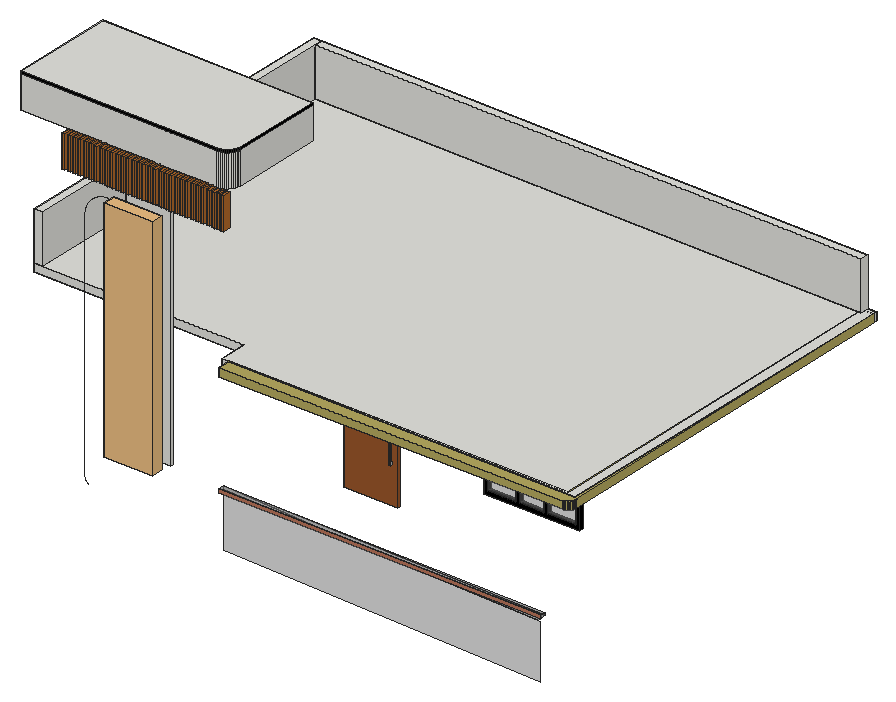
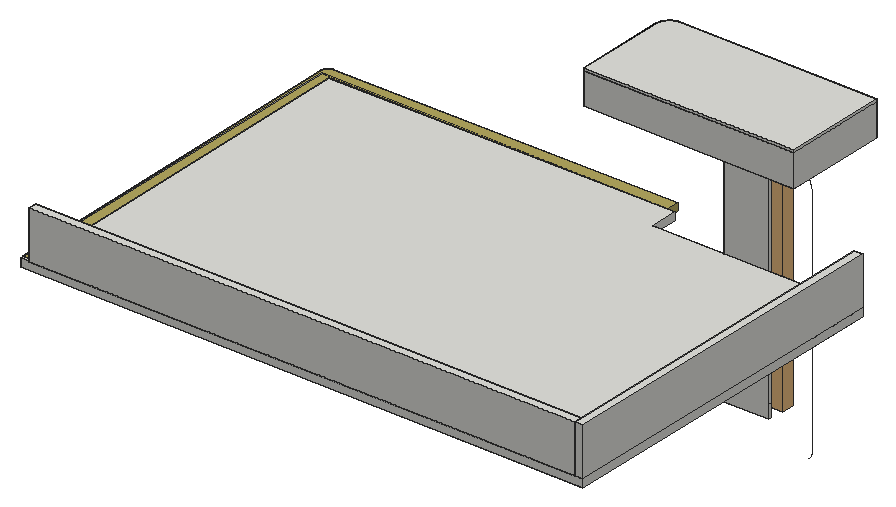
# SketchUp Ruby script. Lengths in inches.
U = 1.inch
M = Sketchup.active_model
def pt(a) = Geom::Point3d.new(a.map { |v| v * U })
def face(e, loops, mat)
  f = e.add_face(loops[0].map { |a| pt(a) })
  loops[1..].each { |l| e.add_face(l.map { |a| pt(a) }).erase! }
  f.material = f.back_material = mat if mat
  f
end
# faces: each face lists its corners as indices into pts; further lists are holes
def faces(e, pts, list, mat = nil) = list.each { |f| face(e, (f[0].is_a?(Array) ? f : [f]).map { |l| l.map { |i| pts[i] } }, mat) }
# xy, xz, yz: faces in a plane at the given z, y or x. An outline is a flat list of corners, or four numbers for a rectangle; further outlines are holes
def ring(l) = l.size == 4 ? [[l[0], l[1]], [l[2], l[1]], [l[2], l[3]], [l[0], l[3]]] : l.each_slice(2).to_a
def flat(e, list, mat, &to3) = list.each { |f| face(e, (f[0].is_a?(Array) ? f : [f]).map { |l| ring(l).map { |u, v| to3.(u, v) } }, mat) }
def xy(e, z, list, mat = nil) = flat(e, list, mat) { |x, y| [x, y, z] }
def xz(e, y, list, mat = nil) = flat(e, list, mat) { |x, z| [x, y, z] }
def yz(e, x, list, mat = nil) = flat(e, list, mat) { |y, z| [x, y, z] }
def lines(e, pts, list) = list.each { |a, b| e.add_line(pt(pts[a]), pt(pts[b])) }
# prism: a flat outline (further loops are holes) pulled along v
def prism(e, loops, v, mat = nil)
  f = face(e, loops, mat); d = Geom::Vector3d.new(v.map { |x| x * U })
  f.pushpull(f.normal.samedirection?(d) ? d.length : -d.length)
end
def box(e, o, s, mat = nil) = prism(e, [[o, [o[0] + s[0], o[1], o[2]], [o[0] + s[0], o[1] + s[1], o[2]], [o[0], o[1] + s[1], o[2]]]], [0, 0, s[2]], mat)
def at(x, y, z, deg = 0) = Geom::Transformation.translation(pt([x, y, z])) * Geom::Transformation.rotation(ORIGIN, Z_AXIS, deg.degrees)
def axes(o, x, y, z) = Geom::Transformation.new([*x, 0, *y, 0, *z, 0, *pt(o).to_a, 1])
def part(name) = M.definitions.add(name)
# library, detail: a bought-in or finely detailed component or shape, given as its bounding box
def library(name, o, s) = part(name).tap { |d| box(d.entities, o, s) }
def detail(e, o, s) = box(e.add_group.entities, o, s)
def put(e, d, t, mat = nil) = e.add_instance(d, t).tap { |i| i.material = mat if mat }
def group(e, t, mat = nil) = e.add_group.tap { |g| g.transformation = t; g.material = mat if mat }.entities
root = M.entities
M.materials.add("[Aluminum]").color = [179, 179, 179]
M.materials.add("[Color M06]").color = [86, 86, 86]
M.materials.add("[Color M09]").color = [0, 0, 0]
M.materials.add("[Metal Rusted]").color = [184, 117, 91]
M.materials.add("[Translucent Glass Gray]").color = [128, 128, 128]
M.materials["[Translucent Glass Gray]"].alpha = 0.5
M.materials.add("[Wood Bamboo]").color = [177, 105, 43]
M.materials.add("[Wood Board Cork]").color = [181, 169, 96]
M.materials.add("[Wood Cherry Original]").color = [152, 86, 42]
c1 = part("Group\#8")
box(c1.entities,[0,-2,0],[40,2,76])
c2 = part("Group\#13")
prism(c2.entities,[[[1.25,1.5,24.92],[1.25,1.5,26.5625],[1.25,0,26.5625],[1.25,0,0],[1.25,1.5,0],[1.25,1.5,1.64],[1.25,0.64,1.64],[1.25,0.64,24.92]]],[-1.25,0,0])
c3 = part("Group\#3")
prism(c3.entities,[[[0,3,0],[0,3,48],[72,3,48],[72,3,0]],[[24,3,3],[24,3,45],[3,3,45],[3,3,3]],[[69,3,45],[48,3,45],[48,3,3],[69,3,3]],[[45,3,3],[45,3,45],[27,3,45],[27,3,3]]],[0,-3,0])
c4 = part("Group\#6")
xz(c4.entities,0,[[0,0,21,42]])
c5 = part("Group\#5")
xz(c5.entities,0,[[0,0,18,42]])
c6 = part("Group\#4")
xz(c6.entities,0,[[0,0,21,42]])
c7 = part("Group\#33")
box(c7.entities,[0,0,0],[2.28,6,24])
xy(root,366,[[0,94.33,0,171.62,156.72,171.62,156.72,104.31,156.64,103.01,156.38,101.73,155.96,100.49,155.39,99.32,154.66,98.24,153.8,97.26,152.82,96.39,151.73,95.67,150.5625,95.09,149.33,94.67,148.05,94.42,146.75,94.33]])
xy(root,390,[[0,94.33,146.75,94.33,148.05,94.42,149.33,94.67,150.5625,95.09,151.73,95.67,152.82,96.39,153.8,97.26,154.66,98.24,155.39,99.32,155.96,100.49,156.38,101.73,156.64,103.01,156.72,104.31,156.72,171.62,0,171.62]])
xy(root,392,[[0,94.33,146.75,94.33,148.05,94.42,149.33,94.67,150.5625,95.09,151.73,95.67,152.82,96.39,153.8,97.26,154.66,98.24,155.39,99.32,155.96,100.49,156.38,101.73,156.64,103.01,156.72,104.31,156.72,171.62,0,171.62]])
xz(root,94.33,[[0,366,146.75,390]])
xz(root,94.33,[[0,390,146.75,392]],"[Color M09]")
xz(root,171.62,[[0,366,156.72,390],[0,390,156.72,392]])
yz(root,0,[[94.33,366,171.62,390],[94.33,390,171.62,392]])
yz(root,156.72,[[104.31,366,171.62,390]])
yz(root,156.72,[[104.31,390,171.62,392]],"[Color M09]")
p = [[148.05,94.42,390],[146.75,94.33,390],[146.75,94.33,366],[148.05,94.42,366],[149.33,94.67,390],[149.33,94.67,366],
  [150.5625,95.09,390],[150.5625,95.09,366],[151.73,95.67,390],[151.73,95.67,366],[152.82,96.39,390],[152.82,96.39,366],
  [153.8,97.26,390],[153.8,97.26,366],[154.66,98.24,390],[154.66,98.24,366],[155.39,99.32,390],[155.39,99.32,366],
  [155.96,100.49,390],[155.96,100.49,366],[156.38,101.73,390],[156.38,101.73,366],[156.64,103.01,390],[156.64,103.01,366],
  [156.72,104.31,390],[156.72,104.31,366],[148.05,94.42,392],[146.75,94.33,392],[149.33,94.67,392],[150.5625,95.09,392],
  [151.73,95.67,392],[152.82,96.39,392],[153.8,97.26,392],[154.66,98.24,392],[155.39,99.32,392],[155.96,100.49,392],
  [156.38,101.73,392],[156.64,103.01,392],[156.72,104.31,392],[51.2,94.33,132.96],[50.6,94.33,133.37],[50.06,94.33,133.84],
  [49.5625,94.33,134.36],[49.13,94.33,134.94],[48.76,94.33,135.5625],[48.46,94.33,136.22],[48.24,94.33,136.9],[48.01,94.33,138.62],
  [48.01,94.33,312.18],[48.17,94.33,314.5],[48.62,94.33,316.79],[49.37,94.33,319],[50.4,94.33,321.09],[51.7,94.33,323.03],
  [53.23,94.33,324.78],[54.99,94.33,326.32],[56.93,94.33,327.61],[59.02,94.33,328.64],[61.22,94.33,329.39],[63.51,94.33,329.85],
  [65.84,94.33,330]]
faces(root,p,[[0,1,2,3],[4,0,3,5],[6,4,5,7],[8,6,7,9],[10,8,9,11],[12,10,11,13],[14,12,13,15],[16,14,15,17],
  [18,16,17,19],[20,18,19,21],[22,20,21,23],[24,22,23,25]])
faces(root,p,[[1,0,26,27],[0,4,28,26],[4,6,29,28],[6,8,30,29],[8,10,31,30],[10,12,32,31],[12,14,33,32],[14,16,34,33],
  [16,18,35,34],[18,20,36,35],[20,22,37,36],[22,24,38,37]],"[Color M09]")
lines(root,p,[[39,40],[40,41],[41,42],[42,43],[43,44],[44,45],[45,46],[47,48],[47,46],[48,49],[49,50],[50,51],
  [51,52],[52,53],[53,54],[54,55],[55,56],[56,57],[57,58],[58,59],[59,60]])
g1 = group(root,at(162.16,74.66,133.26),"[Translucent Glass Gray]")
xy(g1,40.75,[[241,0.04,241,2.61,0,2.61,0,6.79,104.85,3.86,149.47,2.61],[241,0.04,149.47,2.61,241,2.61],[149.47,2.61,104.85,3.86,241,6.79,241,2.61]])
xy(g1,43.375,[[0,2.61,241,6.79]])
xz(g1,2.61,[[0,40.75,241,43.375]],"[Metal Rusted]")
xz(g1,6.79,[[241,40.75,0,43.375,241,43.375]])
yz(g1,0,[[2.61,40.75,6.79,43.375]])
yz(g1,241,[[2.61,40.75,6.79,43.375]])
p = [[0,6.79,0],[0,6.79,40.75],[104.85,3.86,40.75],[149.47,2.61,40.75],[241,0.04,40.75],[242.54,0,40.75],
  [242.54,0,0],[0,6.79,43.375],[241,6.79,40.75]]
faces(g1,p,[[0,1,2,3,4,5,6],[1,7,2],[8,2,7]])
put(root,c1,at(172.72,182.76,136),"[Wood Cherry Original]")
g2 = group(root,at(69.91,107.39,158.71))
prism(g2,[[[0.09,0,10.1875],[0,0,10.1875],[0,0,171.29],[33.59,0,171.29],[33.59,0,0],[0.09,0,0]]],[0,-2,0])
g3 = group(root,at(67.5,97.33,159.9),"[Color M06]")
detail(g3,[0,-9,0],[36,9,170.1])
g4 = group(root,at(70.5,91.21,163.04),"[Translucent Glass Gray]")
g5 = group(g4,at(0,1,51.96))
xz(g5,0,[[0,0,30,36]])
g6 = group(g4,at(0,0,0))
p = [[0.67,1.1,10.97],[0,1,14.86],[31,0,14.86],[30.34,0.14,10.97],[28.72,0.3,7.38],[26.24,0.47,4.3125],
  [23.08,0.64,1.97],[19.42,0.81,0.5],[15.51,0.95,0],[11.6,1.06,0.5],[7.95,1.13,1.97],[4.78,1.16,4.3125],
  [2.3,1.15,7.38],[0,1,49.96],[31,0,49.96]]
faces(g6,p,[[0,1,2,3,4,5,6,7,8,9,10,11,12],[13,14,2,1]])
g7 = group(g4,at(0,1,89.96))
xz(g7,0,[[0,0,30,36]])
g8 = group(g4,at(0,1,127.96))
xz(g8,0,[[0,0,30,36]])
put(root,c2,at(207.62,179.26,163.75),"[Aluminum]")
put(root,c3,at(276.72,181.39,168),"[Color M09]")
put(root,c4,at(279.72,181.39,171),"[Translucent Glass Gray]")
put(root,c5,at(303.72,181.39,171),"[Translucent Glass Gray]")
put(root,c6,at(324.72,181.39,171),"[Translucent Glass Gray]")
g9 = group(root,at(156.72,177.39,216),"[Wood Board Cork]")
prism(g9,[[[-20,2,0],[216,2,0],[216,11,0],[218,11,0],[218,0,0],[-20,0,0]]],[0,0,12])
g10 = group(root,at(162.16,76.76,252),"[Wood Board Cork]")
prism(g10,[[[259.21,288.86,0],[261.29,8.04,0],[261.25,7.28,0],[261.12,6.53,0],[260.89,5.81,0],[260.58,5.12,0],[260.19,4.49,0],[259.73,3.91,0],[259.2,3.4,0],[258.61,2.98,0],[257.97,2.63,0],[257.3,2.38,0],[256.6,2.23,0],[255.89,2.17,0],[0.07,0,0],[0,9.63,0],[252,11.77,0],[249.95,288.78,0]]],[0,0,6])
g11 = group(root,at(-17.28,179.39,252))
prism(g11,[[[174,-72,0],[17.28,-72,0],[17.28,189,0],[438,189,0],[438,-93.06,0],[174,-93.06,0]]],[0,0,6])
g12 = group(root,at(0,107.39,258))
box(g12,[0,0,0],[6,261,36])
g13 = group(root,at(6,362.39,258))
box(g13,[0,0,0],[408.16,6,36])
put(root,c7,at(36,88.33,342),"[Wood Bamboo]")
put(root,c7,at(40,88.33,342),"[Wood Bamboo]")
put(root,c7,at(44,88.33,342),"[Wood Bamboo]")
put(root,c7,at(48,88.33,342),"[Wood Bamboo]")
put(root,c7,at(52,88.33,342),"[Wood Bamboo]")
put(root,c7,at(56,88.33,342),"[Wood Bamboo]")
put(root,c7,at(60,88.33,342),"[Wood Bamboo]")
put(root,c7,at(64,88.33,342),"[Wood Bamboo]")
put(root,c7,at(68,88.33,342),"[Wood Bamboo]")
put(root,c7,at(72,88.33,342),"[Wood Bamboo]")
put(root,c7,at(76,88.33,342),"[Wood Bamboo]")
put(root,c7,at(80,88.33,342),"[Wood Bamboo]")
put(root,c7,at(84,88.33,342),"[Wood Bamboo]")
put(root,c7,at(88,88.33,342),"[Wood Bamboo]")
put(root,c7,at(92,88.33,342),"[Wood Bamboo]")
put(root,c7,at(96,88.33,342),"[Wood Bamboo]")
put(root,c7,at(100,88.33,342),"[Wood Bamboo]")
put(root,c7,at(104,88.33,342),"[Wood Bamboo]")
put(root,c7,at(108,88.33,342),"[Wood Bamboo]")
put(root,c7,at(112,88.33,342),"[Wood Bamboo]")
put(root,c7,at(116,88.33,342),"[Wood Bamboo]")
put(root,c7,at(120,88.33,342),"[Wood Bamboo]")
put(root,c7,at(124,88.33,342),"[Wood Bamboo]")
put(root,c7,at(128,88.33,342),"[Wood Bamboo]")
put(root,c7,at(132,88.33,342),"[Wood Bamboo]")
put(root,c7,at(136,88.33,342),"[Wood Bamboo]")
put(root,c7,at(140,88.33,342),"[Wood Bamboo]")
put(root,c7,at(144,88.33,342),"[Wood Bamboo]")
put(root,c7,at(148,88.33,342),"[Wood Bamboo]")
put(root,c7,at(151.4375,88.33,342),"[Wood Bamboo]")
put(root,c7,at(154.44,88.33,342),"[Wood Bamboo]")
